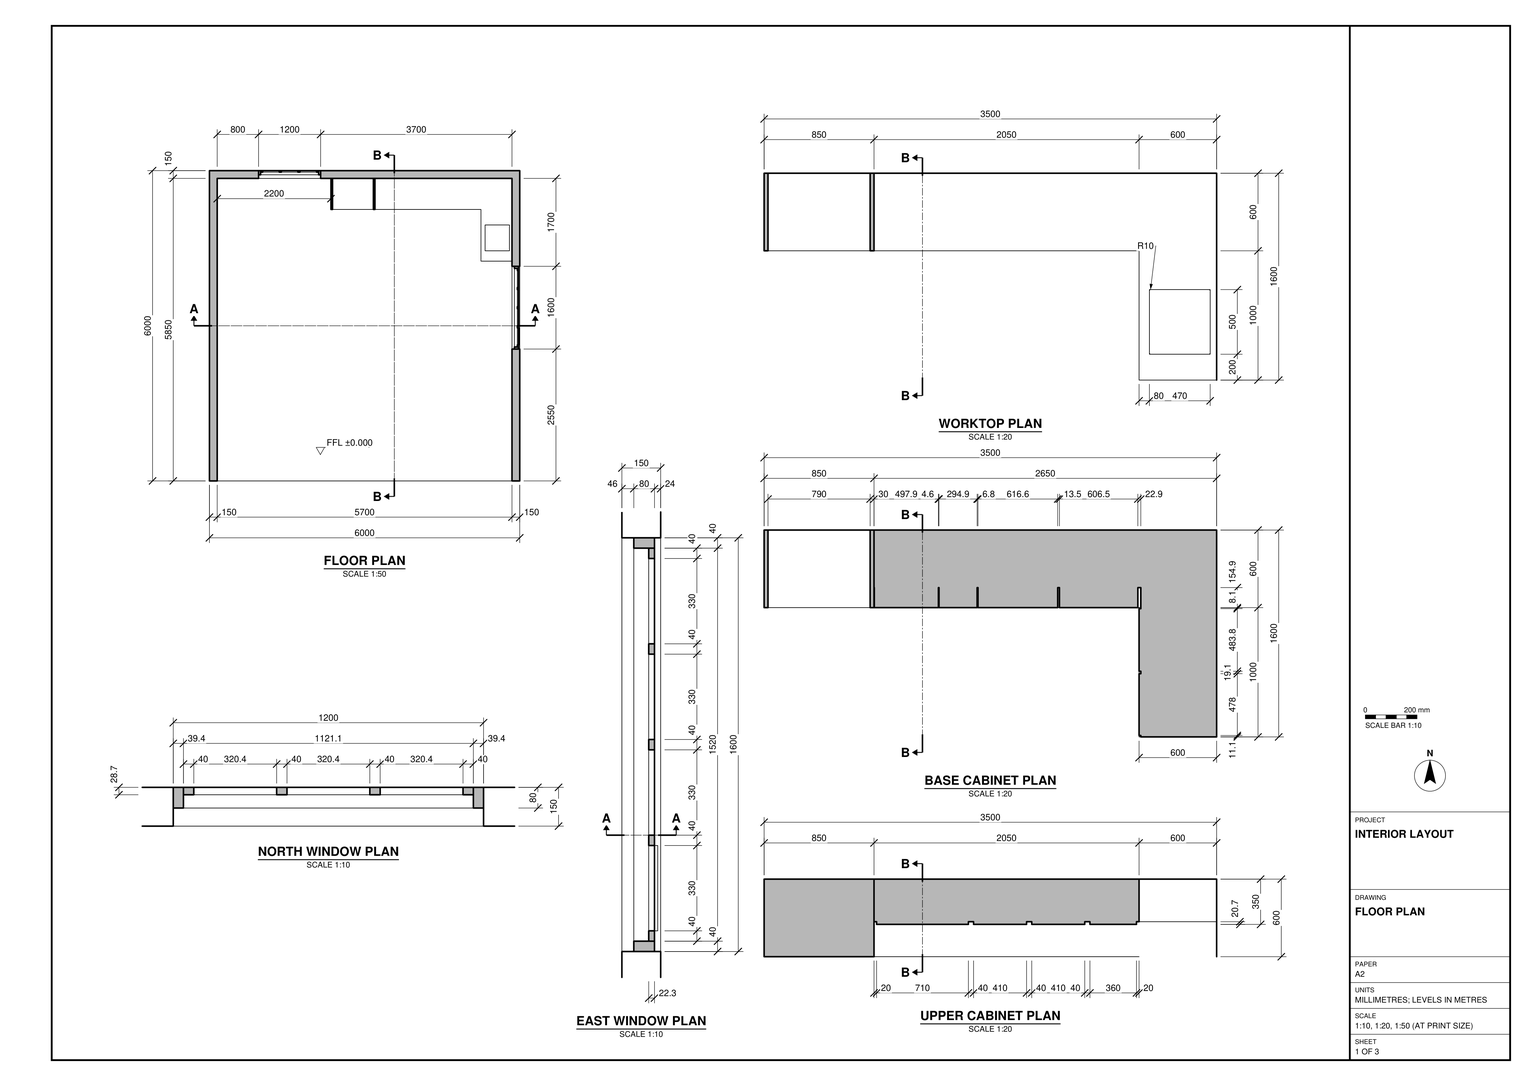
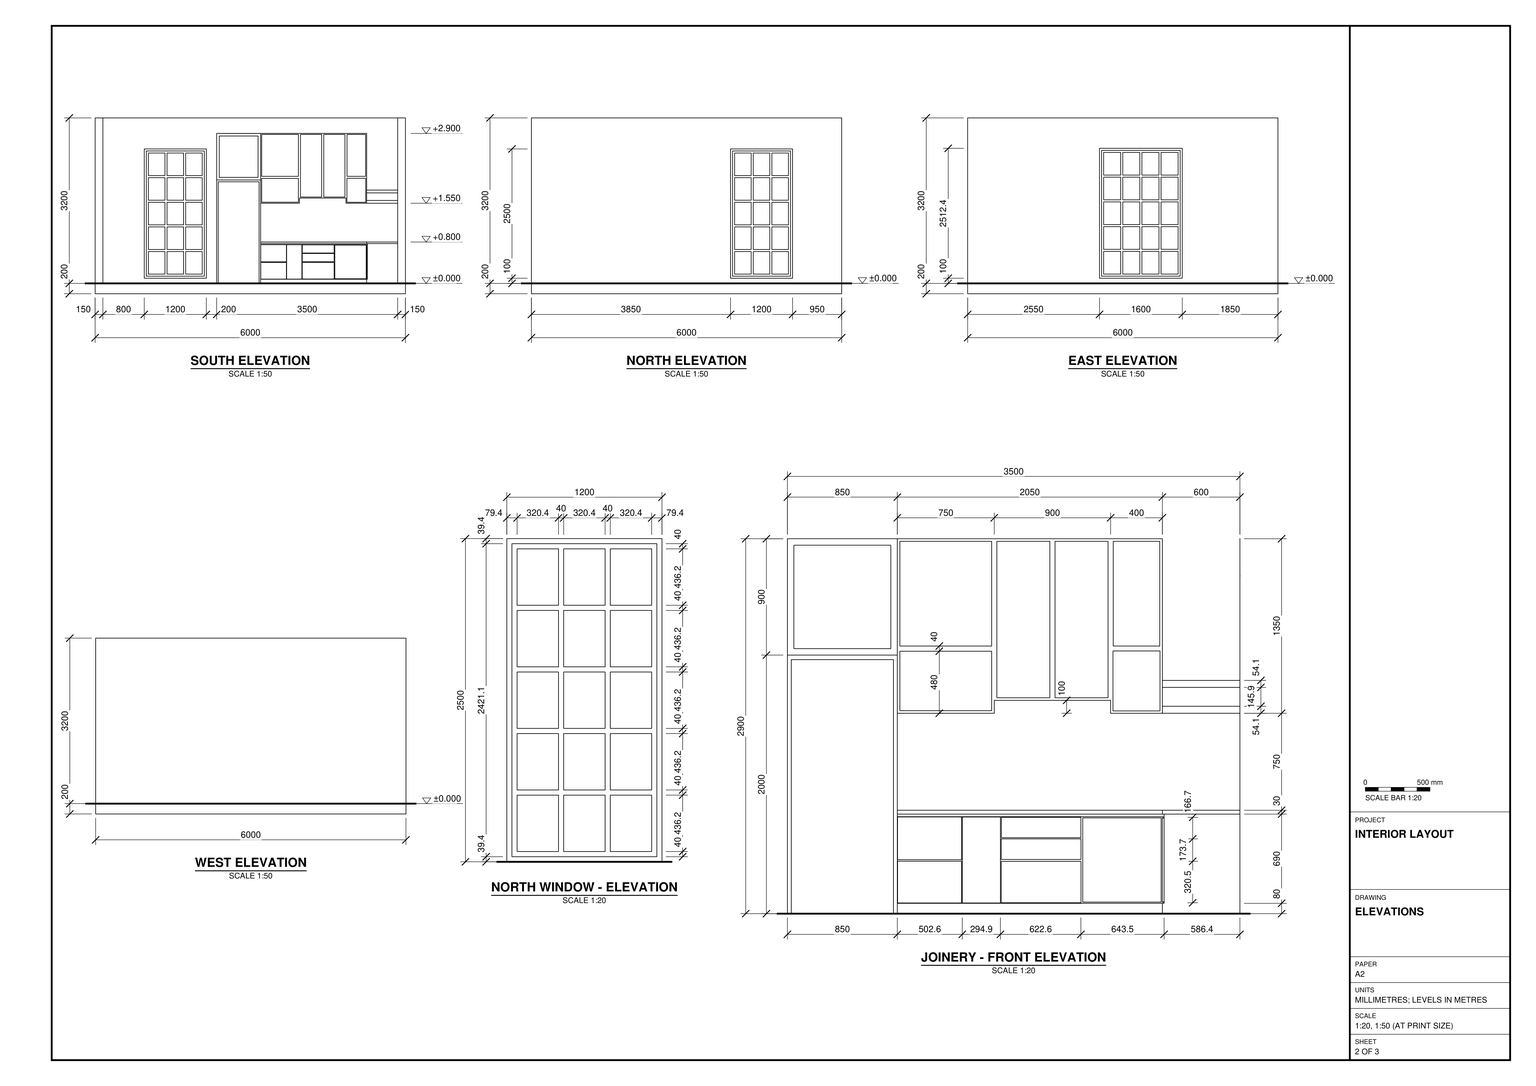
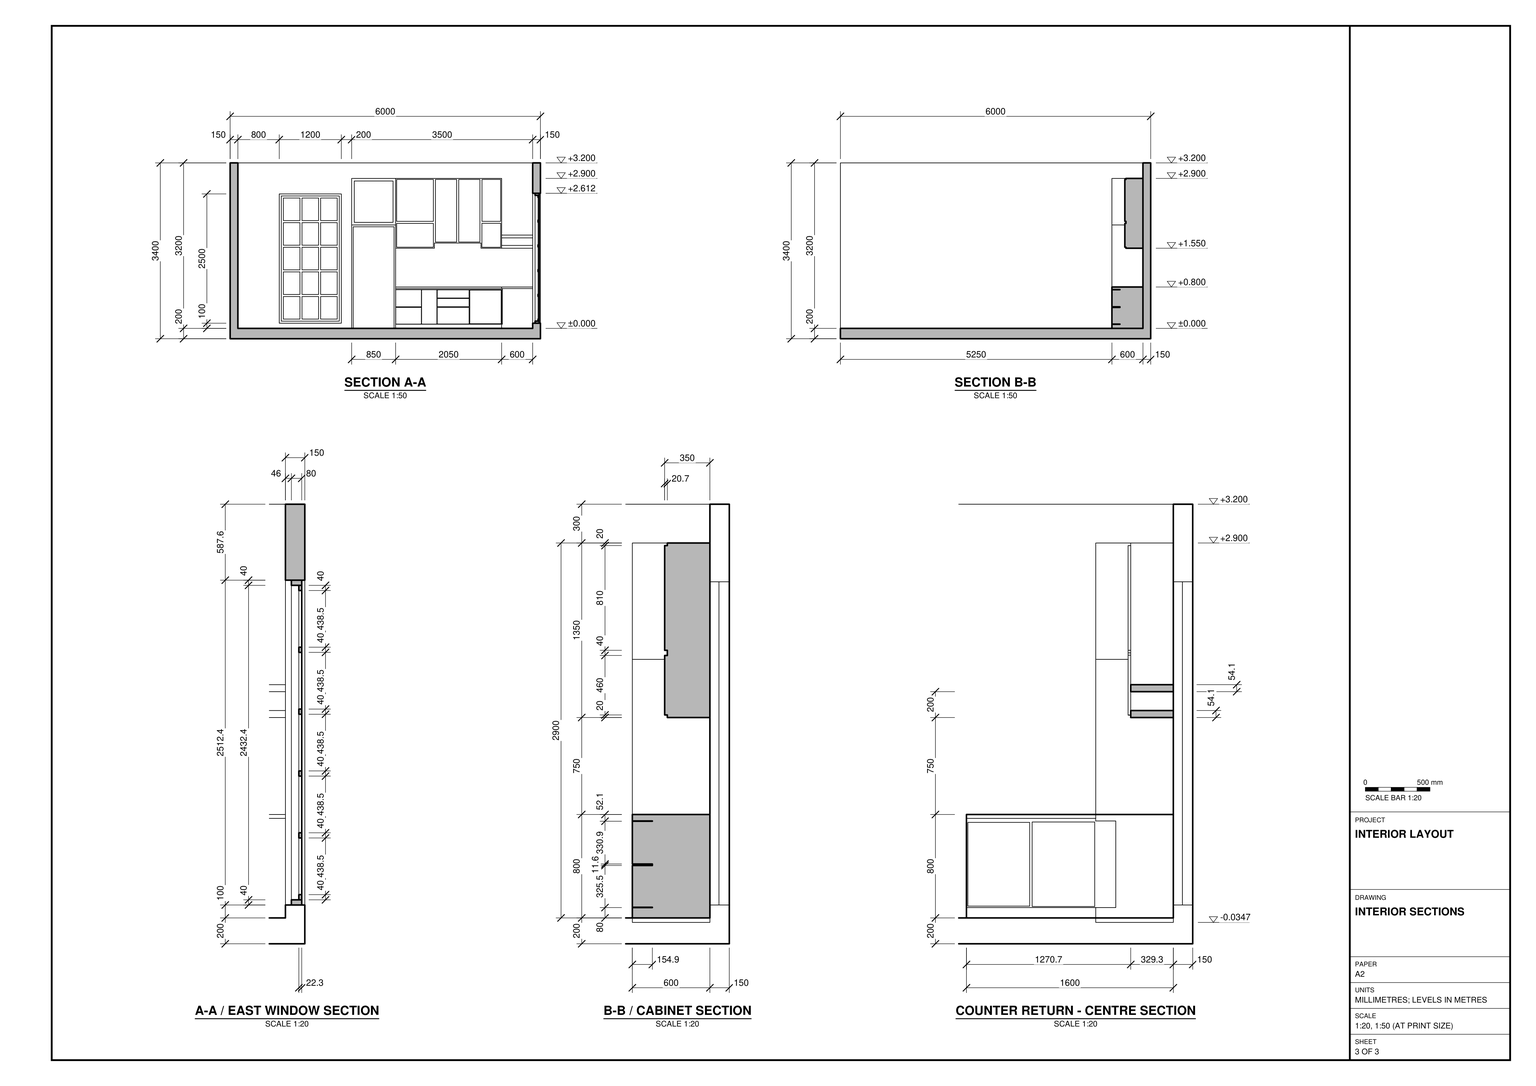
Build the room and its fitted joinery in SketchUp from task_files/diagram_01.pdf. Work in millimetres. The overall model is 6000 mm wide, 6000 mm deep and 3400 mm high. Set the finished floor at 0 mm (±0.000), with the 200 mm slab below it. Build the 150 mm thick north, east and west walls to 3200 mm above the floor. Leave the south side and the top open as shown in the sections.

Set the window units into the north and east wall openings. Use the window details for the frame setbacks, sill positions and glazed pane divisions; the east unit is wider than the north unit. Fit the joinery along the north wall to the right of the north window, with the counter returning along the east wall. Model the tall left bay, the base units on their plinth, the worktop and its rectangular cutout. Follow the front elevation for the drawer and cabinet divisions, the stepped lower edges of the upper cabinets and the short shelves above the return.

Keep the slab, walls, window units and individual joinery pieces in separate groups or components, and use components for repeated parts. Decor and loose items, if used, may be any suitable library components. Save one SketchUp model as output_files/three_sided_room_with_l_shaped_kitchen_joinery.skp.

# SketchUp Ruby script. Lengths in millimetres.
U = 1.mm
M = Sketchup.active_model
def pt(a) = Geom::Point3d.new(a.map { |v| v * U })
def face(e, loops, mat)
  f = e.add_face(loops[0].map { |a| pt(a) })
  loops[1..].each { |l| e.add_face(l.map { |a| pt(a) }).erase! }
  f.material = f.back_material = mat if mat
  f
end
# faces: each face lists its corners as indices into pts; further lists are holes
def faces(e, pts, list, mat = nil) = list.each { |f| face(e, (f[0].is_a?(Array) ? f : [f]).map { |l| l.map { |i| pts[i] } }, mat) }
# xy, xz, yz: faces in a plane at the given z, y or x. An outline is a flat list of corners, or four numbers for a rectangle; further outlines are holes
def ring(l) = l.size == 4 ? [[l[0], l[1]], [l[2], l[1]], [l[2], l[3]], [l[0], l[3]]] : l.each_slice(2).to_a
def flat(e, list, mat, &to3) = list.each { |f| face(e, (f[0].is_a?(Array) ? f : [f]).map { |l| ring(l).map { |u, v| to3.(u, v) } }, mat) }
def xy(e, z, list, mat = nil) = flat(e, list, mat) { |x, y| [x, y, z] }
def xz(e, y, list, mat = nil) = flat(e, list, mat) { |x, z| [x, y, z] }
def yz(e, x, list, mat = nil) = flat(e, list, mat) { |y, z| [x, y, z] }
def lines(e, pts, list) = list.each { |a, b| e.add_line(pt(pts[a]), pt(pts[b])) }
# prism: a flat outline (further loops are holes) pulled along v
def prism(e, loops, v, mat = nil)
  f = face(e, loops, mat); d = Geom::Vector3d.new(v.map { |x| x * U })
  f.pushpull(f.normal.samedirection?(d) ? d.length : -d.length)
end
def box(e, o, s, mat = nil) = prism(e, [[o, [o[0] + s[0], o[1], o[2]], [o[0] + s[0], o[1] + s[1], o[2]], [o[0], o[1] + s[1], o[2]]]], [0, 0, s[2]], mat)
def at(x, y, z, deg = 0) = Geom::Transformation.translation(pt([x, y, z])) * Geom::Transformation.rotation(ORIGIN, Z_AXIS, deg.degrees)
def axes(o, x, y, z) = Geom::Transformation.new([*x, 0, *y, 0, *z, 0, *pt(o).to_a, 1])
def part(name) = M.definitions.add(name)
# library, detail: a bought-in or finely detailed component or shape, given as its bounding box
def library(name, o, s) = part(name).tap { |d| box(d.entities, o, s) }
def detail(e, o, s) = box(e.add_group.entities, o, s)
def put(e, d, t, mat = nil) = e.add_instance(d, t).tap { |i| i.material = mat if mat }
def group(e, t, mat = nil) = e.add_group.tap { |g| g.transformation = t; g.material = mat if mat }.entities
root = M.entities
M.materials.add("[Translucent Glass Gray]").color = [128, 128, 128]
M.materials["[Translucent Glass Gray]"].alpha = 0.5
p = [[5790,4950,1000],[5791.3,4949.9,1000],[5792.6,4949.7,1000],[5793.8,4949.2,1000],[5795,4948.7,1000],[5796.1,4947.9,1000],
  [5797.1,4947.1,1000],[5797.9,4946.1,1000],[5798.7,4945,1000],[5799.2,4943.8,1000],[5799.7,4942.6,1000],[5799.9,4941.3,1000],
  [5800,4940,1000],[5330,4940,1000],[5330.1,4941.3,1000],[5330.3,4942.6,1000],[5330.8,4943.8,1000],[5331.3,4945,1000],
  [5332.1,4946.1,1000],[5332.9,4947.1,1000],[5333.9,4947.9,1000],[5335,4948.7,1000],[5336.2,4949.2,1000],[5337.4,4949.7,1000],
  [5338.7,4949.9,1000],[5340,4950,1000],[5800,4460,1000],[5799.9,4458.7,1000],[5799.7,4457.4,1000],[5799.2,4456.2,1000],
  [5798.7,4455,1000],[5797.9,4453.9,1000],[5797.1,4452.9,1000],[5796.1,4452.1,1000],[5795,4451.3,1000],[5793.8,4450.8,1000],
  [5792.6,4450.3,1000],[5791.3,4450.1,1000],[5790,4450,1000],[5340,4450,1000],[5338.7,4450.1,1000],[5337.4,4450.3,1000],
  [5336.2,4450.8,1000],[5335,4451.3,1000],[5333.9,4452.1,1000],[5332.9,4452.9,1000],[5332.1,4453.9,1000],[5331.3,4455,1000],
  [5330.8,4456.2,1000],[5330.3,4457.4,1000],[5330.1,4458.7,1000],[5330,4460,1000]]
lines(root,p,[[0,1],[1,2],[2,3],[3,4],[4,5],[5,6],[6,7],[7,8],[8,9],[9,10],[10,11],[11,12],
  [13,14],[14,15],[15,16],[16,17],[17,18],[18,19],[19,20],[20,21],[21,22],[22,23],[23,24],[24,25],
  [26,27],[27,28],[28,29],[29,30],[30,31],[31,32],[32,33],[33,34],[34,35],[35,36],[36,37],[37,38],
  [39,40],[40,41],[41,42],[42,43],[43,44],[44,45],[45,46],[46,47],[47,48],[48,49],[49,50],[50,51]])
g1 = group(root,at(0,0,0))
xy(g1,0,[[0,0,6000,6000]])
xy(g1,200,[[150,0,5850,5850]])
xy(g1,300,[[5850,2550,6000,4150],[950,5850,2150,6000]])
xy(g1,339.4,[[989.4,5971.3,2110.6,6000]])
xy(g1,379.4,[[1029.4,5971.3,1349.8,6000],[1389.8,5971.3,1710.2,6000],[1750.2,5971.3,2070.6,6000]])
xy(g1,815.7,[[1029.4,5971.3,1349.8,6000],[1389.8,5971.3,1710.2,6000],[1750.2,5971.3,2070.6,6000]])
xy(g1,855.7,[[1029.4,5971.3,1349.8,6000],[1389.8,5971.3,1710.2,6000],[1750.2,5971.3,2070.6,6000]])
xy(g1,1291.9,[[1029.4,5971.3,1349.8,6000],[1389.8,5971.3,1710.2,6000],[1750.2,5971.3,2070.6,6000]])
xy(g1,1331.9,[[1029.4,5971.3,1349.8,6000],[1389.8,5971.3,1710.2,6000],[1750.2,5971.3,2070.6,6000]])
xy(g1,1768.1,[[1029.4,5971.3,1349.8,6000],[1389.8,5971.3,1710.2,6000],[1750.2,5971.3,2070.6,6000]])
xy(g1,1808.1,[[1029.4,5971.3,1349.8,6000],[1389.8,5971.3,1710.2,6000],[1750.2,5971.3,2070.6,6000]])
xy(g1,2244.3,[[1029.4,5971.3,1349.8,6000],[1389.8,5971.3,1710.2,6000],[1750.2,5971.3,2070.6,6000]])
xy(g1,2284.3,[[1029.4,5971.3,1349.8,6000],[1389.8,5971.3,1710.2,6000],[1750.2,5971.3,2070.6,6000]])
xy(g1,2720.6,[[1029.4,5971.3,1349.8,6000],[1389.8,5971.3,1710.2,6000],[1750.2,5971.3,2070.6,6000]])
xy(g1,2760.6,[[989.4,5971.3,2110.6,6000]])
xy(g1,2800,[[950,5850,2150,6000]])
xy(g1,2812.4,[[5850,2550,6000,4150]])
xy(g1,3400,[[0,0,150,0,150,5850,5850,5850,5850,0,6000,0,6000,6000,0,6000]])
xz(g1,0,[[0,0,6000,0,6000,3400,5850,3400,5850,200,150,200,150,3400,0,3400]])
xz(g1,2550,[[5850,300,6000,2812.4]])
xz(g1,4150,[[5850,300,6000,2812.4]])
xz(g1,5850,[[[150,200,5850,3400],[950,300,2150,2800]]])
xz(g1,5971.3,[[[989.4,339.4,2110.6,2760.6],[1750.2,1331.9,2070.6,1768.1],[1750.2,855.7,2070.6,1291.9],[1029.4,855.7,1349.8,1291.9],[1029.4,1331.9,1349.8,1768.1],[1750.2,379.4,2070.6,815.7],[1029.4,379.4,1349.8,815.7],[1750.2,2284.3,2070.6,2720.6],[1029.4,2284.3,1349.8,2720.6],[1029.4,1808.1,1349.8,2244.3],[1750.2,1808.1,2070.6,2244.3],[1389.8,1331.9,1710.2,1768.1],[1389.8,855.7,1710.2,1291.9],[1389.8,379.4,1710.2,815.7],[1389.8,2284.3,1710.2,2720.6],[1389.8,1808.1,1710.2,2244.3]]])
xz(g1,6000,[[[0,0,6000,3400],[950,300,2150,2800]],[[989.4,339.4,2110.6,2760.6],[1750.2,1331.9,2070.6,1768.1],[1750.2,2284.3,2070.6,2720.6],[1750.2,855.7,2070.6,1291.9],[1750.2,379.4,2070.6,815.7],[1389.8,1331.9,1710.2,1768.1],[1389.8,2284.3,1710.2,2720.6],[1750.2,1808.1,2070.6,2244.3],[1389.8,855.7,1710.2,1291.9],[1029.4,1331.9,1349.8,1768.1],[1389.8,379.4,1710.2,815.7],[1029.4,2284.3,1349.8,2720.6],[1029.4,855.7,1349.8,1291.9],[1389.8,1808.1,1710.2,2244.3],[1029.4,379.4,1349.8,815.7],[1029.4,1808.1,1349.8,2244.3]]])
xz(g1,6000,[[1029.4,379.4,1349.8,815.7],[1389.8,379.4,1710.2,815.7],[1750.2,379.4,2070.6,815.7],[1029.4,855.7,1349.8,1291.9],[1389.8,855.7,1710.2,1291.9],
  [1750.2,855.7,2070.6,1291.9],[1029.4,1331.9,1349.8,1768.1],[1389.8,1331.9,1710.2,1768.1],[1750.2,1331.9,2070.6,1768.1],[1029.4,1808.1,1349.8,2244.3],
  [1389.8,1808.1,1710.2,2244.3],[1750.2,1808.1,2070.6,2244.3],[1029.4,2284.3,1349.8,2720.6],[1389.8,2284.3,1710.2,2720.6],[1750.2,2284.3,2070.6,2720.6]],"[Translucent Glass Gray]")
yz(g1,0,[[0,0,6000,3400]])
yz(g1,150,[[0,200,5850,3400]])
yz(g1,950,[[5850,300,6000,2800]])
yz(g1,989.4,[[5971.3,339.4,6000,2760.6]])
yz(g1,1029.4,[[5971.3,379.4,6000,815.7],[5971.3,855.7,6000,1291.9],[5971.3,1331.9,6000,1768.1],[5971.3,1808.1,6000,2244.3],[5971.3,2284.3,6000,2720.6]])
yz(g1,1349.8,[[5971.3,379.4,6000,815.7],[5971.3,855.7,6000,1291.9],[5971.3,1331.9,6000,1768.1],[5971.3,1808.1,6000,2244.3],[5971.3,2284.3,6000,2720.6]])
yz(g1,1389.8,[[5971.3,379.4,6000,815.7],[5971.3,855.7,6000,1291.9],[5971.3,1331.9,6000,1768.1],[5971.3,1808.1,6000,2244.3],[5971.3,2284.3,6000,2720.6]])
yz(g1,1710.2,[[5971.3,379.4,6000,815.7],[5971.3,855.7,6000,1291.9],[5971.3,1331.9,6000,1768.1],[5971.3,1808.1,6000,2244.3],[5971.3,2284.3,6000,2720.6]])
yz(g1,1750.2,[[5971.3,379.4,6000,815.7],[5971.3,855.7,6000,1291.9],[5971.3,1331.9,6000,1768.1],[5971.3,1808.1,6000,2244.3],[5971.3,2284.3,6000,2720.6]])
yz(g1,2070.6,[[5971.3,379.4,6000,815.7],[5971.3,855.7,6000,1291.9],[5971.3,1331.9,6000,1768.1],[5971.3,1808.1,6000,2244.3],[5971.3,2284.3,6000,2720.6]])
yz(g1,2110.6,[[5971.3,339.4,6000,2760.6]])
yz(g1,2150,[[5850,300,6000,2800]])
yz(g1,5850,[[[0,200,5850,3400],[2550,300,4150,2812.4]]])
yz(g1,6000,[[[0,0,6000,3400],[2550,300,4150,2812.4]]])
g2 = group(g1,at(950,6000,300))
prism(g2,[[[0,-80,0],[1200,-80,0],[1200,-80,2500],[0,-80,2500]],[[39.4,-80,2460.6],[1160.6,-80,2460.6],[1160.6,-80,39.4],[39.4,-80,39.4]]],[0,80,0])
g3 = group(g1,at(6000,2550,300))
prism(g3,[[[-104,1600,2512.4],[-104,1600,0],[-104,0,0],[-104,0,2512.4]],[[-104,1560,2472.4],[-104,40,2472.4],[-104,40,40],[-104,1560,40]]],[80,0,0])
g4 = group(g1,at(5976,2590,340))
xy(g4,0,[[-22.3,0,0,1520]])
xy(g4,40,[[-22.3,40,0,370],[-22.3,410,0,740],[-22.3,780,0,1110],[-22.3,1150,0,1480]])
xy(g4,478.5,[[-22.3,40,0,370],[-22.3,410,0,740],[-22.3,780,0,1110],[-22.3,1150,0,1480]])
xy(g4,518.5,[[-22.3,40,0,370],[0,40,12.5,370],[-22.3,410,0,740],[-22.3,780,0,1110],[-22.3,1150,0,1480]])
xy(g4,956.9,[[-22.3,40,0,370],[0,40,12.5,370],[-22.3,410,0,740],[-22.3,780,0,1110],[-22.3,1150,0,1480]])
xy(g4,996.9,[[-22.3,40,0,370],[-22.3,410,0,740],[-22.3,780,0,1110],[-22.3,1150,0,1480]])
xy(g4,1435.4,[[-22.3,40,0,370],[-22.3,410,0,740],[-22.3,780,0,1110],[-22.3,1150,0,1480]])
xy(g4,1475.4,[[-22.3,40,0,370],[-22.3,410,0,740],[-22.3,780,0,1110],[-22.3,1150,0,1480]])
xy(g4,1913.9,[[-22.3,40,0,370],[-22.3,410,0,740],[-22.3,780,0,1110],[-22.3,1150,0,1480]])
xy(g4,1953.9,[[-22.3,40,0,370],[-22.3,410,0,740],[-22.3,780,0,1110],[-22.3,1150,0,1480]])
xy(g4,2392.4,[[-22.3,40,0,370],[-22.3,410,0,740],[-22.3,780,0,1110],[-22.3,1150,0,1480]])
xy(g4,2432.4,[[-22.3,0,0,1520]])
xz(g4,0,[[-22.3,0,0,2432.4]])
xz(g4,40,[[-22.3,40,0,478.5],[-22.3,518.5,0,956.9],[0,518.5,12.5,956.9],[-22.3,996.9,0,1435.4],[-22.3,1475.4,0,1913.9],
  [-22.3,1953.9,0,2392.4]])
xz(g4,370,[[-22.3,40,0,478.5],[-22.3,518.5,0,956.9],[0,518.5,12.5,956.9],[-22.3,996.9,0,1435.4],[-22.3,1475.4,0,1913.9],
  [-22.3,1953.9,0,2392.4]])
xz(g4,410,[[-22.3,40,0,478.5],[-22.3,518.5,0,956.9],[-22.3,996.9,0,1435.4],[-22.3,1475.4,0,1913.9],[-22.3,1953.9,0,2392.4]])
xz(g4,740,[[-22.3,40,0,478.5],[-22.3,518.5,0,956.9],[-22.3,996.9,0,1435.4],[-22.3,1475.4,0,1913.9],[-22.3,1953.9,0,2392.4]])
xz(g4,780,[[-22.3,40,0,478.5],[-22.3,518.5,0,956.9],[-22.3,996.9,0,1435.4],[-22.3,1475.4,0,1913.9],[-22.3,1953.9,0,2392.4]])
xz(g4,1110,[[-22.3,40,0,478.5],[-22.3,518.5,0,956.9],[-22.3,996.9,0,1435.4],[-22.3,1475.4,0,1913.9],[-22.3,1953.9,0,2392.4]])
xz(g4,1150,[[-22.3,40,0,478.5],[-22.3,518.5,0,956.9],[-22.3,996.9,0,1435.4],[-22.3,1475.4,0,1913.9],[-22.3,1953.9,0,2392.4]])
xz(g4,1480,[[-22.3,40,0,478.5],[-22.3,518.5,0,956.9],[-22.3,996.9,0,1435.4],[-22.3,1475.4,0,1913.9],[-22.3,1953.9,0,2392.4]])
xz(g4,1520,[[-22.3,0,0,2432.4]])
yz(g4,-22.3,[[[0,0,1520,2432.4],[1150,996.9,1480,1435.4],[410,996.9,740,1435.4],[780,996.9,1110,1435.4],[40,996.9,370,1435.4],[1150,1475.4,1480,1913.9],[1150,518.5,1480,956.9],[1150,1953.9,1480,2392.4],[1150,40,1480,478.5],[410,518.5,740,956.9],[410,1475.4,740,1913.9],[780,1475.4,1110,1913.9],[780,518.5,1110,956.9],[40,518.5,370,956.9],[40,1475.4,370,1913.9],[410,1953.9,740,2392.4],[780,1953.9,1110,2392.4],[410,40,740,478.5],[40,1953.9,370,2392.4],[780,40,1110,478.5],[40,40,370,478.5]]])
yz(g4,0,[[[0,0,1520,2432.4],[1150,518.5,1480,956.9],[1150,40,1480,478.5],[1150,1475.4,1480,1913.9],[1150,996.9,1480,1435.4],[1150,1953.9,1480,2392.4],[410,518.5,740,956.9],[410,40,740,478.5],[780,40,1110,478.5],[780,518.5,1110,956.9],[410,996.9,740,1435.4],[410,1475.4,740,1913.9],[780,1475.4,1110,1913.9],[780,996.9,1110,1435.4],[40,40,370,478.5],[40,518.5,370,956.9],[410,1953.9,740,2392.4],[40,996.9,370,1435.4],[40,1475.4,370,1913.9],[780,1953.9,1110,2392.4],[40,1953.9,370,2392.4]]])
yz(g4,0,[[40,40,370,478.5],[410,40,740,478.5],[780,40,1110,478.5],[1150,40,1480,478.5],[410,518.5,740,956.9],
  [780,518.5,1110,956.9],[1150,518.5,1480,956.9],[40,996.9,370,1435.4],[410,996.9,740,1435.4],[780,996.9,1110,1435.4],
  [1150,996.9,1480,1435.4],[40,1475.4,370,1913.9],[410,1475.4,740,1913.9],[780,1475.4,1110,1913.9],[1150,1475.4,1480,1913.9],
  [40,1953.9,370,2392.4],[410,1953.9,740,2392.4],[780,1953.9,1110,2392.4],[1150,1953.9,1480,2392.4]],"[Translucent Glass Gray]")
yz(g4,12.5,[[40,518.5,370,956.9]],"[Translucent Glass Gray]")
g5 = group(g1,at(2350,5250,200))
xy(g5,-34.7,[[30,0,820,600]])
xy(g5,0,[[0,0,30,600],[30,0,820,600],[820,0,850,600]])
xy(g5,1964.8,[[30,0,820,600]])
xz(g5,0,[[30,-34.7,820,0],[0,0,30,0,30,1964.8,820,1964.8,820,0,850,0,850,2000,0,2000]])
xz(g5,600,[[30,-34.7,820,0],[0,0,0,2000,850,2000,850,0,820,0,820,1964.8,30,1964.8,30,0]])
yz(g5,0,[[0,0,600,2000]])
yz(g5,30,[[0,-34.7,600,0],[0,0,600,1964.8]])
yz(g5,820,[[0,-34.7,600,0],[0,0,600,1964.8]])
yz(g5,850,[[0,0,600,2000]])
g6 = group(g5,at(0,0,2000))
xy(g6,-2000,[[2900,-1000,2900,0,850,0,850,600,3500,600,3500,-1000]])
xy(g6,-1920,[[2900,-1000,2913.6,0],[850,0,2913.6,154.9]])
xy(g6,-1917.5,[[852.5,0,1347.5,154.9]])
xy(g6,-1917.4,[[1352.6,0,1647.4,154.9]])
xy(g6,-1915.8,[[1654.2,0,2270.8,154.9]])
xy(g6,-1911.9,[[2900,-491.9,2913.6,-8.1]])
xy(g6,-1910.7,[[2284.3,0,2890.7,154.9]])
xy(g6,-1909,[[2900,-989,2913.6,-511]])
xy(g6,-1595.3,[[1654.2,0,2270.8,154.9]])
xy(g6,-1594.5,[[852.5,0,1347.5,154.9]])
xy(g6,-1582.9,[[852.1,0,1347.9,154.9]])
xy(g6,-1580.8,[[1654.2,0,2270.8,154.9]])
xy(g6,-1421.7,[[1654.2,0,2270.8,154.9]])
xy(g6,-1412.5,[[1655,0,2270,154.9]])
xy(g6,-1261,[[2900,-989,2913.6,-511]])
xy(g6,-1259.3,[[2284.3,0,2890.7,154.9]])
xy(g6,-1258.1,[[2900,-491.9,2913.6,-8.1]])
xy(g6,-1255,[[1655,0,2270,154.9]])
xy(g6,-1252.6,[[1352.6,0,1647.4,154.9]])
xy(g6,-1252.1,[[852.1,0,1347.9,154.9]])
xy(g6,-1250,[[850,0,2913.6,154.9]])
xy(g6,-1230,[[2900,-1000,2913.6,0]])
xy(g6,-1200,[[[2900,-1000,3500,-1000,3500,600,850,600,850,0,2900,0],[2980,-800,3450,-300]],[2980,-800,3450,-300]])
xy(g6,0,[[0,0,850,600]])
xy(g6,900,[[0,0,850,600]])
xz(g6,-1000,[[2900,-2000,3500,-2000,3500,-1230,2913.6,-1230,2913.6,-1920,2900,-1920],[2900,-1230,3500,-1200]])
xz(g6,-989,[[2900,-1909,2913.6,-1261]])
xz(g6,-511,[[2900,-1909,2913.6,-1261]])
xz(g6,-491.9,[[2900,-1911.9,2913.6,-1258.1]])
xz(g6,-8.1,[[2900,-1911.9,2913.6,-1258.1]])
xz(g6,0,[[850,-2000,2900,-1920],[852.5,-1917.5,1347.5,-1594.5],[1352.6,-1917.4,1647.4,-1252.6],[1654.2,-1915.8,2270.8,-1595.3],[2284.3,-1910.7,2890.7,-1259.3],
  [852.1,-1582.9,1347.9,-1252.1],[1654.2,-1580.8,2270.8,-1421.7],[1655,-1412.5,2270,-1255],[850,-1250,2913.6,-1230],[850,-1230,2900,-1200],
  [[0,0,850,900],[50,50,800,850]],[50,50,800,850]])
xz(g6,154.9,[[[850,-1920,2913.6,-1250],[2284.3,-1910.7,2890.7,-1259.3],[1654.2,-1915.8,2270.8,-1595.3],[1352.6,-1917.4,1647.4,-1252.6],[852.1,-1582.9,1347.9,-1252.1],[852.5,-1917.5,1347.5,-1594.5],[1654.2,-1580.8,2270.8,-1421.7],[1655,-1412.5,2270,-1255]]])
xz(g6,600,[[850,-2000,3500,-1200],[0,0,850,900]])
yz(g6,0,[[0,0,600,900]])
yz(g6,850,[[0,-2000,0,-1920,154.9,-1920,154.9,-1250,0,-1250,0,-1200,600,-1200,600,-2000],[0,0,600,900]])
yz(g6,852.1,[[0,-1582.9,154.9,-1252.1]])
yz(g6,852.5,[[0,-1917.5,154.9,-1594.5]])
yz(g6,1347.5,[[0,-1917.5,154.9,-1594.5]])
yz(g6,1347.9,[[0,-1582.9,154.9,-1252.1]])
yz(g6,1352.6,[[0,-1917.4,154.9,-1585],[0,-1585,154.9,-1252.6]])
yz(g6,1647.4,[[0,-1917.4,154.9,-1585],[0,-1585,154.9,-1417.5],[0,-1417.5,154.9,-1252.6]])
yz(g6,1654.2,[[0,-1915.8,154.9,-1595.3],[0,-1580.8,154.9,-1421.7]])
yz(g6,1655,[[0,-1412.5,154.9,-1255]])
yz(g6,2270,[[0,-1412.5,154.9,-1255]])
yz(g6,2270.8,[[0,-1915.8,154.9,-1595.3],[0,-1580.8,154.9,-1421.7]])
yz(g6,2284.3,[[0,-1910.7,154.9,-1259.3]])
yz(g6,2890.7,[[0,-1910.7,154.9,-1259.3]])
yz(g6,2900,[[-1000,-2000,0,-1920],[-491.9,-1911.9,-8.1,-1258.1],[-989,-1909,-511,-1261],[-1000,-1230,0,-1200]])
yz(g6,2913.6,[[[-1000,-1920,-1000,-1230,0,-1230,0,-1250,154.9,-1250,154.9,-1920],[-491.9,-1911.9,-8.1,-1258.1],[-989,-1909,-511,-1261]]])
yz(g6,3500,[[-1000,-2000,600,-1200]])
g7 = group(g6,at(2900,600,-445.9))
box(g7,[0,-329.3,-4.1],[600,329.3,54.1])
box(g7,[0,-329.3,195.9],[600,329.3,54.1])
g8 = group(g5,at(850,600,1550))
xy(g8,0,[[0,-329.3,750,0],[1650,-329.3,2050,0]])
xy(g8,18.1,[[1668.1,-350,2031.9,-329.3]])
xy(g8,20,[[20,-350,730,-329.3]])
xy(g8,100,[[750,-329.3,1650,0]])
xy(g8,120,[[770,-350,1180,-329.3],[1220,-350,1630,-329.3]])
xy(g8,480,[[20,-350,730,-329.3]])
xy(g8,481.9,[[1668.1,-350,2031.9,-329.3]])
xy(g8,520,[[20,-350,730,-329.3],[1670,-350,2030,-329.3]])
xy(g8,1330,[[20,-350,730,-329.3],[770,-350,1180,-329.3],[1220,-350,1630,-329.3],[1670,-350,2030,-329.3]])
xy(g8,1350,[[0,-329.3,2050,0]])
xz(g8,-350,[[1668.1,18.1,2031.9,481.9],[20,20,730,480],[770,120,1180,1330],[1220,120,1630,1330],[20,520,730,1330],
  [1670,520,2030,1330]])
xz(g8,-329.3,[[[0,0,750,0,750,100,1650,100,1650,0,2050,0,2050,1350,0,1350],[20,520,730,1330],[1220,120,1630,1330],[770,120,1180,1330],[20,20,730,480],[1670,520,2030,1330],[1668.1,18.1,2031.9,481.9]]])
xz(g8,0,[[0,0,0,1350,2050,1350,2050,0,1650,0,1650,100,750,100,750,0]])
yz(g8,0,[[-329.3,0,0,450],[-329.3,450,0,1350]])
yz(g8,20,[[-350,20,-329.3,450],[-350,450,-329.3,480],[-350,520,-329.3,1330]])
yz(g8,730,[[-350,20,-329.3,100],[-350,100,-329.3,480],[-350,520,-329.3,1330]])
yz(g8,750,[[-329.3,0,0,100]])
yz(g8,770,[[-350,120,-329.3,500],[-350,500,-329.3,1330]])
yz(g8,1180,[[-350,120,-329.3,1330]])
yz(g8,1220,[[-350,120,-329.3,1330]])
yz(g8,1630,[[-350,120,-329.3,500],[-350,500,-329.3,1330]])
yz(g8,1650,[[-329.3,0,0,100]])
yz(g8,1668.1,[[-350,18.1,-329.3,100],[-350,100,-329.3,481.9]])
yz(g8,1670,[[-350,520,-329.3,1330]])
yz(g8,2030,[[-350,520,-329.3,1330]])
yz(g8,2031.9,[[-350,18.1,-329.3,481.9]])
yz(g8,2050,[[-329.3,0,0,1350]])
